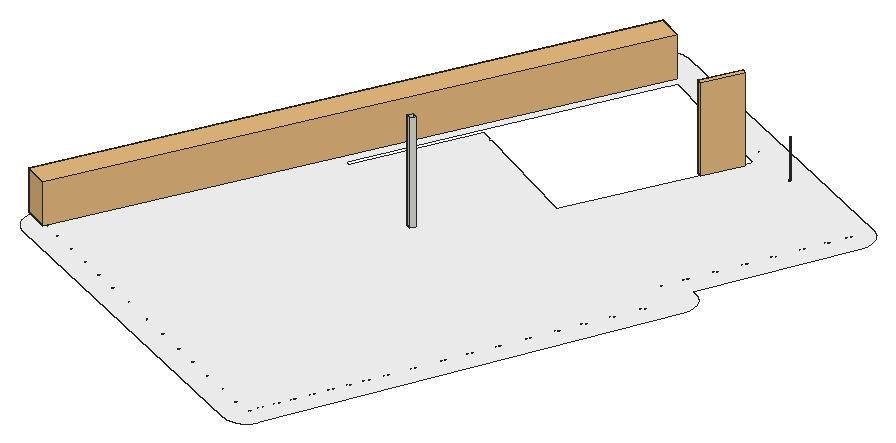
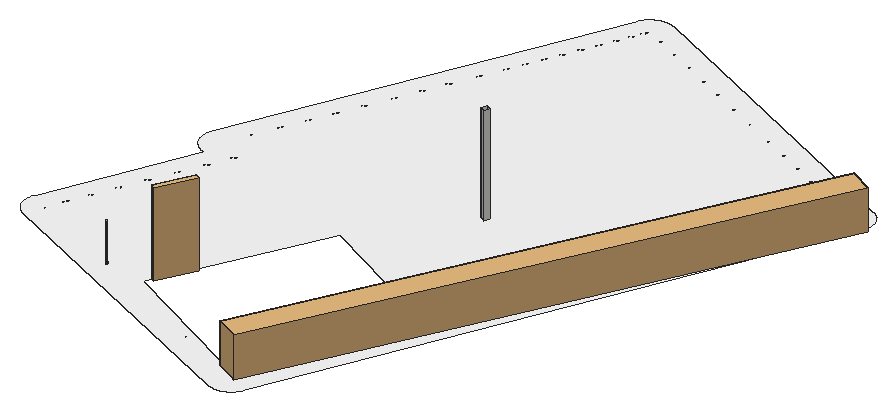
# SketchUp Ruby script. Lengths in inches.
U = 1.inch
M = Sketchup.active_model
def pt(a) = Geom::Point3d.new(a.map { |v| v * U })
def face(e, loops, mat)
  f = e.add_face(loops[0].map { |a| pt(a) })
  loops[1..].each { |l| e.add_face(l.map { |a| pt(a) }).erase! }
  f.material = f.back_material = mat if mat
  f
end
# faces: each face lists its corners as indices into pts; further lists are holes
def faces(e, pts, list, mat = nil) = list.each { |f| face(e, (f[0].is_a?(Array) ? f : [f]).map { |l| l.map { |i| pts[i] } }, mat) }
# xy, xz, yz: faces in a plane at the given z, y or x. An outline is a flat list of corners, or four numbers for a rectangle; further outlines are holes
def ring(l) = l.size == 4 ? [[l[0], l[1]], [l[2], l[1]], [l[2], l[3]], [l[0], l[3]]] : l.each_slice(2).to_a
def flat(e, list, mat, &to3) = list.each { |f| face(e, (f[0].is_a?(Array) ? f : [f]).map { |l| ring(l).map { |u, v| to3.(u, v) } }, mat) }
def xy(e, z, list, mat = nil) = flat(e, list, mat) { |x, y| [x, y, z] }
def xz(e, y, list, mat = nil) = flat(e, list, mat) { |x, z| [x, y, z] }
def yz(e, x, list, mat = nil) = flat(e, list, mat) { |y, z| [x, y, z] }
def lines(e, pts, list) = list.each { |a, b| e.add_line(pt(pts[a]), pt(pts[b])) }
# prism: a flat outline (further loops are holes) pulled along v
def prism(e, loops, v, mat = nil)
  f = face(e, loops, mat); d = Geom::Vector3d.new(v.map { |x| x * U })
  f.pushpull(f.normal.samedirection?(d) ? d.length : -d.length)
end
def box(e, o, s, mat = nil) = prism(e, [[o, [o[0] + s[0], o[1], o[2]], [o[0] + s[0], o[1] + s[1], o[2]], [o[0], o[1] + s[1], o[2]]]], [0, 0, s[2]], mat)
def at(x, y, z, deg = 0) = Geom::Transformation.translation(pt([x, y, z])) * Geom::Transformation.rotation(ORIGIN, Z_AXIS, deg.degrees)
def axes(o, x, y, z) = Geom::Transformation.new([*x, 0, *y, 0, *z, 0, *pt(o).to_a, 1])
def part(name) = M.definitions.add(name)
# library, detail: a bought-in or finely detailed component or shape, given as its bounding box
def library(name, o, s) = part(name).tap { |d| box(d.entities, o, s) }
def detail(e, o, s) = box(e.add_group.entities, o, s)
def put(e, d, t, mat = nil) = e.add_instance(d, t).tap { |i| i.material = mat if mat }
def group(e, t, mat = nil) = e.add_group.tap { |g| g.transformation = t; g.material = mat if mat }.entities
root = M.entities
M.materials.add("[Color_000]").color = [255, 255, 255]
c1 = library("Group\#120",[0,0,0],[510.78,23.69,36.98])
c2 = library("porta 4",[0.2,-5.42,1.33],[46.55,4.72,83.21])
xy(root,321.267,[[[841.443,516.19,840.136,516.256,838.836,516.408,837.549,516.645,836.28,516.965,835.035,517.367,833.818,517.85,548.6875,642.033,547.506,642.595,546.363,643.233,545.264,643.944,544.214,644.725,543.217,645.574,542.279,646.485,541.401,647.457,540.589,648.483,539.846,649.56,539.176,650.684,538.579,651.849,538.061,653.051,537.622,654.284,537.265,655.543,536.991,656.823,536.801,658.118,536.696,659.422,536.677,660.731,536.743,662.038,536.895,663.338,537.132,664.625,537.452,665.894,537.854,667.139,538.337,668.356,741.172,1134.074,741.733,1135.256,742.371,1136.399,743.082,1137.498,743.863,1138.547,744.712,1139.544,745.623,1140.483,746.595,1141.36,747.621,1142.172,748.699,1142.915,749.822,1143.586,750.987,1144.182,752.189,1144.7,753.422,1145.139,754.681,1145.497,755.961,1145.771,757.256,1145.961,758.56,1146.065,759.869,1146.084,761.176,1146.018,762.476,1145.866,763.763,1145.63,765.032,1145.31,766.278,1144.907,767.494,1144.424,1030.621,1029.824,1031.803,1029.263,1032.946,1028.625,1034.045,1027.914,1035.095,1027.133,1036.091,1026.284,1037.03,1025.372,1037.908,1024.401,1038.719,1023.375,1039.462,1022.297,1040.133,1021.174,1040.729,1020.008,1041.248,1018.807,1041.687,1017.574,1042.044,1016.315,1042.318,1015.035,1042.508,1013.74,1042.613,1012.435,1042.632,1011.127,1042.565,1009.82,1042.414,1008.52,1042.177,1007.233,1041.857,1005.964,1041.455,1004.718,1040.971,1003.502,985.468,876.064,989.136,874.467,990.318,873.905,991.461,873.268,992.56,872.556,993.609,871.775,994.606,870.927,995.545,870.015,996.422,869.044,997.234,868.017,997.977,866.94,998.648,865.816,999.244,864.651,999.762,863.449,1000.201,862.216,1000.558,860.957,1000.833,859.677,1001.022,858.382,1001.127,857.078,1001.146,855.769,1001.08,854.462,1000.928,853.162,1000.692,851.875,1000.372,850.606,999.969,849.361,999.486,848.144,860.141,528.201,859.579,527.019,858.942,525.876,858.231,524.777,857.449,523.727,856.601,522.73,855.689,521.792,854.718,520.914,853.691,520.102,852.614,519.359,851.49,518.688,850.325,518.092,849.123,517.574,847.89,517.135,846.631,516.778,845.352,516.504,844.057,516.314,842.752,516.209],[671.218,867.453,718.811,965.468,728.334,960.844,728.204,960.454,728.18,960.044,728.262,959.641,728.446,959.274,728.719,958.966,729.0625,958.74,729.453,958.61,729.863,958.586,730.266,958.668,730.633,958.852,730.941,959.125,731.167,959.469,826.624,913.117,831.121,910.933,881.579,1014.847,896.797,1046.187,897.141,1046.896,900.471,1053.753,783.663,1110.472,780.622,1104.208,780.366,1103.681,780.333,1103.614,714.314,967.652,666.72,869.637],[843.13,535.199,843.291,535.232,843.4375,535.305,843.561,535.415,843.651,535.552,843.703,535.708,843.713,535.872,843.68,536.033,843.606,536.18,843.547,536.247,843.722,536.189,844.132,536.165,844.535,536.247,844.587,536.273,844.902,536.431,845.21,536.704,845.436,537.047,845.566,537.4375,845.59,537.848,845.508,538.251,845.323,538.618,845.051,538.926,844.707,539.152,844.645,539.173,847.388,545.47,847.716,545.361,848.127,545.337,848.529,545.419,848.897,545.603,849.204,545.876,849.431,546.219,849.56,546.61,849.585,547.02,849.502,547.423,849.318,547.79,849.045,548.098,848.702,548.324,848.64,548.345,852.607,557.453,852.935,557.344,853.346,557.32,853.748,557.402,854.116,557.587,854.423,557.859,854.65,558.203,854.78,558.593,854.804,559.003,854.721,559.406,854.537,559.773,854.264,560.081,853.921,560.307,853.859,560.328,858.009,569.857,858.337,569.748,858.748,569.723,859.151,569.806,859.518,569.99,859.826,570.263,860.052,570.606,860.182,570.996,860.206,571.407,860.123,571.809,859.939,572.177,859.666,572.484,859.323,572.711,859.261,572.731,864.264,584.217,864.592,584.108,865.002,584.083,865.405,584.166,865.772,584.35,866.08,584.623,866.306,584.966,866.436,585.356,866.46,585.767,866.378,586.169,866.194,586.537,865.921,586.844,865.577,587.071,865.515,587.091,870.373,598.244,870.701,598.135,871.111,598.11,871.514,598.193,871.882,598.377,872.189,598.65,872.415,598.993,872.545,599.383,872.569,599.794,872.487,600.196,872.303,600.564,872.03,600.871,871.687,601.098,871.625,601.118,876.101,611.396,876.116,611.386,876.506,611.257,876.916,611.232,877.319,611.315,877.687,611.499,877.994,611.772,878.22,612.115,878.35,612.505,878.374,612.916,878.292,613.318,878.108,613.686,877.835,613.993,877.492,614.22,877.351,614.266,882.234,625.478,882.294,625.411,882.637,625.184,883.027,625.055,883.437,625.03,883.84,625.113,884.208,625.297,884.515,625.57,884.741,625.913,884.871,626.303,884.895,626.714,884.813,627.116,884.629,627.484,884.356,627.791,884.013,628.018,883.622,628.147,883.402,628.16,888.589,640.071,888.918,639.961,889.328,639.937,889.731,640.02,890.098,640.204,890.406,640.477,890.632,640.82,890.762,641.21,890.786,641.62,890.704,642.023,890.519,642.391,890.247,642.698,889.903,642.924,889.841,642.945,897.491,660.509,897.819,660.4,898.23,660.376,898.633,660.459,899,660.643,899.308,660.916,899.534,661.259,899.664,661.649,899.688,662.059,899.605,662.462,899.421,662.83,899.148,663.137,898.805,663.363,898.743,663.384,907.436,683.344,907.765,683.235,908.175,683.21,908.578,683.293,908.945,683.477,909.253,683.75,909.479,684.093,909.609,684.483,909.633,684.894,909.55,685.296,909.366,685.664,909.093,685.971,908.75,686.198,908.688,686.218,916.156,703.365,916.484,703.255,916.895,703.231,917.297,703.314,917.665,703.498,917.972,703.771,918.199,704.114,918.328,704.504,918.353,704.914,918.27,705.317,918.086,705.685,917.813,705.992,917.47,706.218,917.408,706.239,925.387,724.56,925.716,724.451,926.126,724.427,926.529,724.51,926.896,724.694,927.204,724.967,927.43,725.31,927.56,725.7,927.584,726.11,927.501,726.513,927.317,726.881,927.044,727.188,926.701,727.414,926.639,727.435,935.3125,747.349,935.641,747.24,936.051,747.215,936.454,747.298,936.821,747.482,937.129,747.755,937.355,748.098,937.485,748.488,937.509,748.899,937.426,749.301,937.242,749.669,936.969,749.976,936.626,750.203,936.564,750.223,944.632,768.748,944.647,768.738,945.037,768.608,945.448,768.584,945.85,768.666,946.218,768.85,946.525,769.123,946.752,769.467,946.881,769.857,946.906,770.267,946.823,770.67,946.639,771.037,946.366,771.345,946.023,771.571,945.882,771.618,953.644,789.44,953.917,789.133,954.261,788.907,954.651,788.777,955.061,788.753,955.464,788.835,955.831,789.019,956.139,789.292,956.365,789.636,956.495,790.026,956.519,790.436,956.437,790.839,956.252,791.206,955.979,791.514,955.636,791.74,955.246,791.87,954.836,791.894,954.701,791.867,962.796,810.452,963.124,810.343,963.534,810.319,963.937,810.401,964.305,810.585,964.612,810.858,964.838,811.202,964.968,811.592,964.993,812.002,964.91,812.405,964.726,812.772,964.453,813.08,964.11,813.306,964.048,813.327,972.962,833.794,973.29,833.685,973.7,833.66,974.103,833.743,974.471,833.927,974.778,834.2,975.004,834.543,975.134,834.933,975.159,835.344,975.076,835.746,974.892,836.114,974.619,836.421,974.276,836.648,974.214,836.668,973.886,836.777,973.475,836.802,973.072,836.719,972.705,836.535,972.397,836.262,972.171,835.919,972.041,835.529,972.017,835.118,972.1,834.716,972.284,834.348,972.557,834.041,972.9,833.814,972.962,833.794,964.048,813.327,963.72,813.436,963.309,813.46,962.906,813.377,962.539,813.193,962.231,812.92,962.005,812.577,961.875,812.187,961.851,811.777,961.934,811.374,962.118,811.006,962.391,810.699,962.734,810.473,962.796,810.452,954.701,791.867,954.433,791.811,954.065,791.627,953.758,791.354,953.532,791.011,953.402,790.621,953.378,790.211,953.46,789.808,953.644,789.44,945.882,771.618,945.633,771.701,945.222,771.725,944.82,771.643,944.452,771.458,944.145,771.185,943.918,770.842,943.789,770.452,943.764,770.042,943.847,769.639,944.031,769.272,944.304,768.964,944.632,768.748,936.564,750.223,936.236,750.332,935.826,750.357,935.423,750.274,935.055,750.09,934.748,749.817,934.522,749.474,934.392,749.084,934.368,748.673,934.45,748.271,934.634,747.903,934.907,747.596,935.251,747.369,935.3125,747.349,926.639,727.435,926.311,727.544,925.901,727.568,925.498,727.486,925.13,727.302,924.823,727.029,924.597,726.686,924.467,726.295,924.443,725.885,924.525,725.482,924.709,725.115,924.982,724.807,925.325,724.581,925.387,724.56,917.408,706.239,917.08,706.348,916.669,706.373,916.267,706.29,915.899,706.106,915.592,705.833,915.365,705.49,915.236,705.1,915.211,704.689,915.294,704.287,915.478,703.919,915.751,703.612,916.094,703.385,916.156,703.365,908.688,686.218,908.36,686.327,907.95,686.352,907.547,686.269,907.179,686.085,906.872,685.812,906.646,685.469,906.516,685.079,906.492,684.668,906.574,684.266,906.758,683.898,907.031,683.591,907.374,683.364,907.436,683.344,898.743,663.384,898.415,663.493,898.005,663.517,897.602,663.435,897.234,663.251,896.927,662.978,896.701,662.635,896.571,662.245,896.546,661.834,896.629,661.431,896.813,661.064,897.086,660.756,897.429,660.53,897.491,660.509,889.841,642.945,889.513,643.054,889.103,643.079,888.7,642.996,888.333,642.812,888.025,642.539,887.799,642.196,887.669,641.806,887.645,641.395,887.727,640.992,887.911,640.625,888.184,640.317,888.528,640.091,888.589,640.071,883.402,628.16,883.212,628.172,882.809,628.089,882.442,627.905,882.134,627.632,881.908,627.289,881.778,626.899,881.754,626.488,881.837,626.086,882.021,625.718,882.234,625.478,877.351,614.266,877.101,614.349,876.691,614.374,876.288,614.291,875.921,614.107,875.613,613.834,875.387,613.491,875.257,613.101,875.233,612.69,875.316,612.288,875.5,611.92,875.773,611.613,876.101,611.396,871.625,601.118,871.296,601.227,870.886,601.252,870.483,601.169,870.116,600.985,869.808,600.712,869.582,600.369,869.452,599.979,869.428,599.568,869.511,599.166,869.695,598.798,869.968,598.491,870.311,598.264,870.373,598.244,865.515,587.091,865.187,587.2,864.777,587.225,864.374,587.142,864.007,586.958,863.699,586.685,863.473,586.342,863.343,585.952,863.319,585.541,863.401,585.139,863.585,584.771,863.858,584.464,864.202,584.237,864.264,584.217,859.261,572.731,858.933,572.84,858.523,572.865,858.12,572.782,857.752,572.598,857.445,572.325,857.219,571.982,857.089,571.592,857.065,571.181,857.147,570.779,857.331,570.411,857.604,570.104,857.947,569.877,858.009,569.857,853.859,560.328,853.531,560.437,853.121,560.461,852.718,560.379,852.35,560.195,852.043,559.922,851.817,559.578,851.687,559.188,851.662,558.778,851.745,558.375,851.929,558.008,852.202,557.7,852.545,557.474,852.607,557.453,848.64,548.345,848.312,548.454,847.902,548.478,847.499,548.395,847.131,548.211,846.824,547.938,846.597,547.595,846.468,547.205,846.443,546.795,846.526,546.392,846.71,546.024,846.983,545.717,847.326,545.491,847.388,545.47,844.645,539.173,844.317,539.282,843.907,539.306,843.504,539.223,843.137,539.039,842.829,538.766,842.603,538.423,842.473,538.033,842.449,537.623,842.517,537.289,842.531,537.22,842.715,536.852,842.988,536.545,843.133,536.45,843.039,536.455,842.878,536.422,842.731,536.349,842.608,536.239,842.518,536.102,842.466,535.946,842.456,535.782,842.489,535.621,842.563,535.474,842.672,535.351,842.809,535.26,842.846,535.248,842.965,535.208],[827.381,539.408,827.783,539.491,828.151,539.675,828.458,539.948,828.685,540.291,828.705,540.352,828.815,540.681,828.839,541.092,828.756,541.494,828.572,541.862,828.299,542.169,827.956,542.396,827.566,542.525,827.156,542.55,826.753,542.467,826.385,542.283,826.078,542.01,825.851,541.667,825.83,541.603,809.71,548.624,809.819,548.953,809.844,549.363,809.761,549.766,809.577,550.133,809.304,550.441,808.961,550.667,808.571,550.797,808.16,550.821,807.758,550.738,807.39,550.554,807.083,550.281,806.856,549.938,806.836,549.876,788.49,557.867,788.599,558.195,788.623,558.605,788.54,559.008,788.356,559.375,788.083,559.683,787.74,559.909,787.35,560.039,786.94,560.063,786.537,559.981,786.169,559.797,785.862,559.524,785.636,559.18,785.615,559.118,767.513,567.002,767.623,567.33,767.647,567.741,767.564,568.144,767.38,568.511,767.107,568.819,766.764,569.045,766.374,569.175,765.964,569.199,765.561,569.116,765.193,568.932,764.886,568.659,764.66,568.316,764.639,568.254,747.167,575.864,747.276,576.192,747.301,576.602,747.218,577.005,747.034,577.373,746.761,577.68,746.418,577.906,746.028,578.036,745.617,578.06,745.215,577.978,744.847,577.794,744.54,577.521,744.313,577.178,744.293,577.116,724.462,585.753,724.571,586.081,724.596,586.491,724.513,586.894,724.329,587.261,724.056,587.569,723.713,587.795,723.323,587.925,722.912,587.949,722.509,587.867,722.142,587.682,721.834,587.41,721.608,587.066,721.588,587.004,701.946,595.559,702.055,595.887,702.08,596.297,701.997,596.7,701.813,597.068,701.54,597.375,701.197,597.601,700.807,597.731,700.396,597.756,699.994,597.673,699.626,597.489,699.319,597.216,699.092,596.873,699.072,596.811,675.709,606.986,675.818,607.314,675.843,607.724,675.76,608.127,675.576,608.495,675.303,608.802,674.96,609.028,674.57,609.158,674.159,609.183,673.757,609.1,673.389,608.916,673.082,608.643,672.855,608.3,672.835,608.238,653.14,616.816,653.249,617.144,653.273,617.554,653.19,617.957,653.006,618.324,652.733,618.632,652.39,618.858,652,618.988,651.59,619.012,651.187,618.93,650.819,618.746,650.512,618.473,650.286,618.129,650.265,618.067,633.494,625.372,633.603,625.7,633.628,626.11,633.545,626.513,633.361,626.881,633.088,627.188,632.745,627.414,632.355,627.544,631.944,627.568,631.542,627.486,631.174,627.302,630.867,627.029,630.64,626.686,630.62,626.624,613.859,633.924,613.968,634.252,613.992,634.662,613.91,635.065,613.726,635.432,613.453,635.74,613.109,635.966,612.719,636.096,612.309,636.12,611.906,636.038,611.539,635.854,611.231,635.581,611.005,635.237,610.984,635.175,593.863,642.632,593.972,642.961,593.996,643.371,593.914,643.774,593.73,644.141,593.457,644.449,593.113,644.675,592.723,644.805,592.313,644.829,591.91,644.746,591.543,644.5625,591.235,644.289,591.009,643.946,590.988,643.884,574.051,651.261,574.16,651.589,574.184,652,574.101,652.402,573.917,652.77,573.644,653.077,573.301,653.304,572.911,653.434,572.501,653.458,572.098,653.375,571.73,653.191,571.423,652.918,571.197,652.575,571.176,652.513,558.139,658.191,558.27,658.307,558.496,658.65,558.626,659.04,558.65,659.451,558.568,659.854,558.383,660.221,558.111,660.529,557.767,660.755,557.377,660.885,556.967,660.909,556.564,660.826,556.197,660.642,555.901,660.38,555.889,660.369,555.663,660.026,555.533,659.636,555.529,659.561,555.509,659.226,555.591,658.823,555.775,658.455,555.88,658.337,556.048,658.148,556.392,657.922,556.782,657.792,557.192,657.767,557.595,657.85,557.962,658.034,558.139,658.191,571.176,652.513,571.067,652.185,571.043,651.775,571.125,651.372,571.309,651.004,571.582,650.697,571.925,650.471,572.316,650.341,572.726,650.316,573.129,650.399,573.496,650.583,573.804,650.856,574.03,651.199,574.051,651.261,590.988,643.884,590.879,643.556,590.855,643.146,590.9375,642.743,591.121,642.375,591.394,642.068,591.738,641.842,592.128,641.712,592.538,641.6875,592.941,641.77,593.308,641.954,593.616,642.227,593.842,642.57,593.863,642.632,610.984,635.175,610.875,634.847,610.851,634.437,610.933,634.034,611.117,633.667,611.39,633.359,611.734,633.133,612.124,633.003,612.534,632.979,612.937,633.061,613.304,633.245,613.612,633.518,613.838,633.862,613.859,633.924,630.62,626.624,630.511,626.295,630.486,625.885,630.569,625.482,630.753,625.115,631.026,624.807,631.369,624.581,631.759,624.451,632.17,624.427,632.572,624.51,632.94,624.694,633.247,624.967,633.474,625.31,633.494,625.372,650.265,618.067,650.156,617.739,650.132,617.329,650.214,616.926,650.398,616.559,650.671,616.251,651.014,616.025,651.405,615.895,651.815,615.871,652.218,615.953,652.585,616.138,652.893,616.41,653.119,616.754,653.14,616.816,672.835,608.238,672.726,607.91,672.701,607.499,672.784,607.096,672.968,606.729,673.241,606.421,673.584,606.195,673.974,606.065,674.385,606.041,674.787,606.124,675.155,606.308,675.462,606.581,675.689,606.924,675.709,606.986,699.072,596.811,698.962,596.483,698.938,596.072,699.021,595.67,699.205,595.302,699.478,594.994,699.821,594.768,700.211,594.638,700.621,594.614,701.024,594.697,701.392,594.881,701.699,595.154,701.925,595.497,701.946,595.559,721.588,587.004,721.478,586.676,721.454,586.266,721.537,585.863,721.721,585.496,721.994,585.188,722.337,584.962,722.727,584.832,723.137,584.808,723.54,584.89,723.908,585.074,724.215,585.347,724.441,585.691,724.462,585.753,744.293,577.116,744.184,576.787,744.159,576.377,744.242,575.974,744.426,575.607,744.699,575.299,745.042,575.073,745.432,574.943,745.843,574.919,746.245,575.002,746.613,575.186,746.92,575.459,747.147,575.802,747.167,575.864,764.639,568.254,764.53,567.926,764.505,567.516,764.588,567.113,764.772,566.745,765.045,566.438,765.388,566.212,765.778,566.082,766.189,566.057,766.592,566.14,766.959,566.324,767.267,566.597,767.493,566.94,767.513,567.002,785.615,559.118,785.506,558.79,785.482,558.38,785.564,557.977,785.748,557.61,786.021,557.302,786.364,557.076,786.755,556.946,787.165,556.922,787.568,557.004,787.935,557.188,788.243,557.461,788.469,557.805,788.49,557.867,806.836,549.876,806.726,549.548,806.702,549.138,806.785,548.735,806.969,548.367,807.242,548.06,807.585,547.834,807.975,547.704,808.385,547.68,808.788,547.762,809.156,547.946,809.463,548.219,809.69,548.5625,809.71,548.624,825.83,541.603,825.722,541.277,825.697,540.866,825.78,540.464,825.964,540.096,826.237,539.789,826.58,539.5625,826.97,539.433],[961.916,866.707,962.319,866.79,962.686,866.974,962.994,867.247,963.22,867.59,963.35,867.98,963.374,868.391,963.291,868.793,963.107,869.161,962.834,869.469,962.491,869.695,962.429,869.715,970.135,887.408,970.463,887.298,970.873,887.274,971.276,887.357,971.644,887.541,971.951,887.814,972.177,888.157,972.307,888.547,972.332,888.957,972.249,889.36,972.065,889.728,971.792,890.035,971.449,890.261,971.387,890.282,979.763,909.514,980.091,909.405,980.502,909.381,980.904,909.464,981.272,909.648,981.579,909.921,981.806,910.264,981.935,910.654,981.96,911.064,981.877,911.467,981.693,911.835,981.42,912.142,981.077,912.368,981.015,912.389,989.406,931.655,989.734,931.545,990.144,931.521,990.547,931.604,990.915,931.788,991.222,932.061,991.448,932.404,991.578,932.794,991.602,933.204,991.52,933.607,991.336,933.975,991.063,934.282,990.72,934.508,990.658,934.529,999.023,953.736,999.351,953.627,999.761,953.602,1000.164,953.685,1000.532,953.869,1000.839,954.142,1001.065,954.485,1001.195,954.875,1001.219,955.286,1001.137,955.688,1000.953,956.056,1000.68,956.363,1000.337,956.59,1000.275,956.61,1008.368,975.194,1008.696,975.085,1009.107,975.06,1009.51,975.143,1009.877,975.327,1010.185,975.6,1010.411,975.943,1010.541,976.333,1010.565,976.744,1010.482,977.146,1010.298,977.514,1010.025,977.821,1009.682,978.048,1009.62,978.068,1016.34,993.498,1016.669,993.389,1017.079,993.365,1017.482,993.447,1017.849,993.631,1018.157,993.904,1018.383,994.248,1018.513,994.638,1018.537,995.048,1018.455,995.451,1018.27,995.818,1017.998,996.126,1017.654,996.352,1017.592,996.373,1023.808,1010.645,1023.955,1011.013,1023.974,1011.074,1023.991,1011.073,1024.394,1011.156,1024.762,1011.34,1025.069,1011.613,1025.295,1011.956,1025.425,1012.346,1025.45,1012.756,1025.367,1013.159,1025.183,1013.527,1024.91,1013.834,1024.567,1014.061,1024.177,1014.19,1023.766,1014.215,1023.363,1014.132,1023.238,1014.069,1022.996,1013.948,1022.688,1013.675,1022.538,1013.446,1022.462,1013.332,1022.396,1013.133,1022.332,1012.942,1022.308,1012.531,1022.32,1012.471,1022.391,1012.129,1022.575,1011.761,1022.704,1011.616,1022.848,1011.454,1023.191,1011.227,1023.581,1011.098,1023.974,1011.074,1023.955,1011.013,1023.808,1010.645,1017.592,996.373,1017.264,996.482,1016.854,996.506,1016.451,996.424,1016.084,996.24,1015.776,995.967,1015.55,995.623,1015.42,995.233,1015.396,994.823,1015.478,994.42,1015.662,994.053,1015.935,993.745,1016.279,993.519,1016.34,993.498,1009.62,978.068,1009.292,978.177,1008.882,978.202,1008.479,978.119,1008.111,977.935,1007.804,977.662,1007.578,977.319,1007.448,976.929,1007.423,976.518,1007.506,976.116,1007.69,975.748,1007.963,975.441,1008.306,975.214,1008.368,975.194,1000.275,956.61,999.946,956.719,999.536,956.744,999.133,956.661,998.766,956.477,998.458,956.204,998.232,955.861,998.102,955.471,998.078,955.06,998.161,954.658,998.345,954.29,998.618,953.983,998.961,953.756,999.023,953.736,990.658,934.529,990.329,934.638,989.919,934.663,989.516,934.58,989.149,934.396,988.841,934.123,988.615,933.78,988.485,933.39,988.461,932.979,988.544,932.577,988.728,932.209,989.001,931.901,989.344,931.675,989.406,931.655,981.015,912.389,980.687,912.498,980.276,912.522,979.874,912.44,979.506,912.256,979.199,911.983,978.972,911.64,978.843,911.249,978.818,910.839,978.901,910.436,979.085,910.069,979.358,909.761,979.701,909.535,979.763,909.514,971.387,890.282,971.059,890.391,970.648,890.416,970.245,890.333,969.878,890.149,969.57,889.876,969.344,889.533,969.214,889.143,969.19,888.732,969.273,888.33,969.457,887.962,969.73,887.655,970.073,887.428,970.135,887.408,962.429,869.715,962.101,869.825,961.691,869.849,961.288,869.766,960.92,869.582,960.613,869.309,960.387,868.966,960.257,868.576,960.233,868.166,960.315,867.763,960.499,867.395,960.772,867.088,961.115,866.862,961.177,866.841,961.506,866.732],[765.123,821.855,767.291,826.319,762.793,828.503,760.626,824.039],[554.814,657.808,555.217,657.891,555.585,658.075,555.88,658.337,555.892,658.348,556.118,658.691,556.231,659.029,556.248,659.081,556.273,659.492,556.19,659.894,556.006,660.262,555.901,660.38,555.733,660.569,555.39,660.796,555.343,660.811,555,660.925,554.589,660.95,554.186,660.867,553.819,660.683,553.511,660.41,553.285,660.067,553.155,659.677,553.131,659.266,553.214,658.864,553.398,658.496,553.671,658.189,554.014,657.962,554.404,657.833],[824.098,1097.975,824.501,1098.058,824.868,1098.242,825.176,1098.515,825.402,1098.858,825.423,1098.92,824.56,1099.296,824.604,1099.427,824.614,1099.591,824.581,1099.752,824.507,1099.899,824.398,1100.022,824.261,1100.113,824.105,1100.165,823.94,1100.175,823.779,1100.142,823.632,1100.068,823.509,1099.959,823.419,1099.821,823.411,1099.797,822.548,1100.172,822.439,1099.844,822.415,1099.434,822.497,1099.031,822.681,1098.663,822.954,1098.356,823.298,1098.13,823.6875,1098],[1015.608,1014.567,1016.011,1014.65,1016.378,1014.834,1016.686,1015.107,1016.912,1015.45,1016.932,1015.512,1016.07,1015.888,1016.114,1016.019,1016.124,1016.183,1016.09,1016.344,1016.017,1016.491,1015.908,1016.614,1015.77,1016.705,1015.614,1016.757,1015.45,1016.766,1015.289,1016.733,1015.142,1016.66,1015.019,1016.55,1014.929,1016.413,1014.92,1016.388,1014.058,1016.764,1013.949,1016.436,1013.924,1016.025,1014.007,1015.623,1014.191,1015.255,1014.464,1014.948,1014.807,1014.721,1015.197,1014.592],[871.348,1077.397,871.751,1077.479,872.118,1077.663,872.426,1077.936,872.652,1078.28,872.673,1078.342,871.81,1078.717,871.854,1078.848,871.864,1079.013,871.831,1079.174,871.757,1079.321,871.648,1079.444,871.511,1079.534,871.355,1079.586,871.19,1079.596,871.029,1079.563,870.882,1079.489,870.759,1079.38,870.669,1079.243,870.661,1079.218,869.798,1079.593,869.689,1079.265,869.665,1078.855,869.747,1078.452,869.931,1078.085,870.204,1077.777,870.548,1077.551,870.9375,1077.421],[893.192,1067.883,893.595,1067.966,893.962,1068.15,894.27,1068.423,894.496,1068.766,894.517,1068.828,893.654,1069.203,893.698,1069.335,893.708,1069.499,893.675,1069.66,893.601,1069.807,893.492,1069.93,893.354,1070.02,893.198,1070.072,893.034,1070.082,892.873,1070.049,892.726,1069.975,892.603,1069.866,892.513,1069.729,892.504,1069.704,891.642,1070.08,891.533,1069.752,891.509,1069.341,891.591,1068.938,891.775,1068.571,892.048,1068.263,892.391,1068.037,892.782,1067.907],[916.821,1057.592,917.223,1057.675,917.591,1057.859,917.898,1058.132,918.125,1058.475,918.145,1058.537,917.283,1058.912,917.327,1059.044,917.336,1059.208,917.303,1059.369,917.23,1059.516,917.121,1059.639,916.983,1059.729,916.827,1059.781,916.663,1059.791,916.502,1059.758,916.355,1059.684,916.232,1059.575,916.142,1059.438,916.133,1059.413,915.271,1059.789,915.162,1059.461,915.137,1059.05,915.22,1058.647,915.404,1058.28,915.677,1057.972,916.02,1057.746,916.41,1057.616],[938.054,1048.344,938.457,1048.427,938.824,1048.611,939.132,1048.884,939.358,1049.227,939.379,1049.289,938.516,1049.665,938.56,1049.796,938.57,1049.96,938.537,1050.121,938.463,1050.268,938.354,1050.391,938.217,1050.482,938.061,1050.534,937.896,1050.543,937.735,1050.51,937.588,1050.437,937.465,1050.327,937.375,1050.19,937.367,1050.165,936.504,1050.541,936.395,1050.213,936.371,1049.802,936.453,1049.4,936.637,1049.032,936.91,1048.725,937.254,1048.498,937.644,1048.369],[957.437,1039.902,957.84,1039.985,958.208,1040.169,958.515,1040.442,958.741,1040.785,958.762,1040.847,957.9,1041.223,957.943,1041.354,957.953,1041.518,957.92,1041.679,957.846,1041.826,957.737,1041.949,957.6,1042.04,957.444,1042.092,957.28,1042.101,957.118,1042.068,956.971,1041.995,956.848,1041.885,956.758,1041.748,956.75,1041.723,955.887,1042.099,955.778,1041.771,955.754,1041.36,955.837,1040.958,956.021,1040.59,956.294,1040.283,956.637,1040.056,957.027,1039.927],[800.488,1108.258,800.891,1108.341,801.258,1108.525,801.566,1108.798,801.792,1109.141,801.813,1109.203,800.95,1109.579,800.994,1109.71,801.004,1109.874,800.971,1110.035,800.897,1110.182,800.788,1110.305,800.651,1110.396,800.495,1110.448,800.331,1110.457,800.169,1110.424,800.022,1110.351,799.899,1110.242,799.809,1110.104,799.801,1110.079,798.938,1110.455,798.829,1110.127,798.805,1109.716,798.887,1109.314,799.072,1108.946,799.344,1108.639,799.6875,1108.412,800.078,1108.283],[996.475,1022.9,996.878,1022.983,997.246,1023.167,997.553,1023.44,997.779,1023.783,997.8,1023.845,996.938,1024.22,996.981,1024.352,996.991,1024.516,996.958,1024.677,996.884,1024.824,996.775,1024.947,996.638,1025.037,996.482,1025.089,996.318,1025.099,996.157,1025.066,996.01,1024.992,995.887,1024.883,995.796,1024.746,995.788,1024.721,994.926,1025.097,994.816,1024.769,994.792,1024.358,994.875,1023.955,995.059,1023.588,995.332,1023.28,995.675,1023.054,996.065,1022.924],[975.893,1031.864,976.296,1031.947,976.663,1032.131,976.971,1032.404,977.197,1032.747,977.218,1032.809,976.355,1033.185,976.399,1033.316,976.409,1033.48,976.376,1033.641,976.302,1033.788,976.193,1033.911,976.056,1034.002,975.9,1034.054,975.735,1034.063,975.574,1034.03,975.427,1033.957,975.304,1033.847,975.214,1033.71,975.206,1033.685,974.343,1034.061,974.234,1033.733,974.21,1033.322,974.292,1032.92,974.476,1032.552,974.749,1032.245,975.093,1032.018,975.483,1031.889],[848.682,1087.269,849.084,1087.351,849.452,1087.535,849.759,1087.808,849.986,1088.151,850.006,1088.213,849.144,1088.589,849.1875,1088.72,849.197,1088.884,849.164,1089.045,849.091,1089.192,848.982,1089.315,848.844,1089.406,848.688,1089.458,848.524,1089.468,848.363,1089.435,848.216,1089.361,848.093,1089.252,848.002,1089.114,847.994,1089.09,847.132,1089.465,847.023,1089.137,846.998,1088.727,847.081,1088.324,847.265,1087.956,847.538,1087.649,847.881,1087.423,848.271,1087.293],[760.58,1127.161,760.587,1127.184,760.612,1127.594,760.529,1127.997,760.345,1128.364,760.072,1128.672,759.729,1128.898,759.339,1129.028,758.929,1129.052,758.526,1128.969,758.158,1128.785,757.851,1128.512,757.624,1128.169,757.495,1127.779,757.483,1127.574,757.641,1127.607,758.052,1127.582,758.414,1127.462,758.423,1127.6,758.474,1127.756,758.565,1127.894,758.688,1128.003,758.835,1128.077,758.996,1128.11,759.16,1128.1,759.316,1128.048,759.454,1127.957,759.563,1127.834,759.636,1127.6875,759.669,1127.526,759.667,1127.48,759.716,1127.475,759.806,1127.458,759.895,1127.436,759.983,1127.407,760.351,1127.261],[776.144,1118.861,776.547,1118.944,776.914,1119.128,777.222,1119.401,777.448,1119.744,777.469,1119.806,776.606,1120.181,776.598,1120.156,776.508,1120.019,776.385,1119.91,776.238,1119.836,776.077,1119.803,775.912,1119.813,775.756,1119.865,775.619,1119.956,775.51,1120.078,775.436,1120.226,775.403,1120.387,775.413,1120.551,775.457,1120.682,774.594,1121.058,774.485,1120.729,774.461,1120.319,774.543,1119.916,774.728,1119.549,775,1119.241,775.344,1119.015,775.734,1118.885],[982.5,856.655,982.661,856.688,982.808,856.762,982.931,856.871,983.022,857.008,983.074,857.164,983.083,857.328,983.05,857.489,982.977,857.636,982.868,857.759,982.73,857.85,982.574,857.902,982.41,857.912,982.249,857.878,982.136,857.822,982.102,857.805,981.979,857.696,981.888,857.558,981.837,857.402,981.834,857.354,981.827,857.238,981.86,857.077,981.934,856.93,982.004,856.851,982.043,856.807,982.18,856.717,982.336,856.665,982.449,856.658],[1022.108,1012.412,1022.269,1012.445,1022.32,1012.471,1022.416,1012.519,1022.539,1012.628,1022.63,1012.766,1022.681,1012.922,1022.686,1013.006,1022.691,1013.086,1022.658,1013.247,1022.584,1013.394,1022.538,1013.446,1022.475,1013.517,1022.338,1013.607,1022.182,1013.659,1022.018,1013.669,1021.857,1013.636,1021.71,1013.562,1021.611,1013.474,1021.587,1013.453,1021.496,1013.316,1021.444,1013.16,1021.435,1012.996,1021.468,1012.835,1021.541,1012.6875,1021.65,1012.565,1021.788,1012.474,1021.944,1012.422],[980.642,856.926,980.803,856.959,980.916,857.016,980.95,857.033,981.073,857.142,981.164,857.279,981.216,857.435,981.225,857.599,981.217,857.642,981.192,857.76,981.119,857.907,981.049,857.986,981.01,858.03,980.872,858.121,980.716,858.173,980.552,858.183,980.391,858.15,980.244,858.076,980.236,858.069,980.121,857.967,980.03,857.829,979.979,857.673,979.969,857.509,980.002,857.348,980.075,857.201,980.185,857.078,980.322,856.988,980.478,856.936],[759.154,1125.911,759.3125,1125.943,759.325,1126.148,759.242,1126.551,759.09,1126.854,759.086,1126.853,758.922,1126.863,758.766,1126.915,758.629,1127.005,758.541,1127.103,758.534,1127.097,758.47,1127.031,758.411,1126.961,758.356,1126.888,758.306,1126.811,758.262,1126.731,758.16,1126.516,758.166,1126.512,758.276,1126.389,758.349,1126.242,758.382,1126.081,758.381,1126.056,758.743,1125.935],[776.606,1120.181,776.65,1120.3125,776.66,1120.477,776.627,1120.638,776.553,1120.785,776.444,1120.908,776.307,1120.998,776.151,1121.05,775.987,1121.06,775.825,1121.027,775.678,1120.953,775.555,1120.844,775.465,1120.707,775.457,1120.682],[800.421,1109.201,800.582,1109.234,800.729,1109.307,800.852,1109.417,800.942,1109.554,800.95,1109.579,799.801,1110.079,799.757,1109.948,799.747,1109.784,799.78,1109.623,799.854,1109.476,799.963,1109.353,800.1,1109.262,800.256,1109.211],[1015.54,1015.51,1015.701,1015.543,1015.848,1015.616,1015.971,1015.726,1016.062,1015.863,1016.07,1015.888,1014.92,1016.388,1014.877,1016.257,1014.867,1016.093,1014.9,1015.932,1014.974,1015.785,1015.083,1015.662,1015.22,1015.571,1015.376,1015.519],[871.28,1078.339,871.442,1078.372,871.589,1078.446,871.712,1078.555,871.802,1078.692,871.81,1078.717,870.661,1079.218,870.617,1079.087,870.607,1078.922,870.64,1078.761,870.714,1078.614,870.823,1078.491,870.96,1078.401,871.116,1078.349],[996.408,1023.842,996.569,1023.875,996.716,1023.949,996.839,1024.058,996.929,1024.196,996.938,1024.22,995.788,1024.721,995.744,1024.59,995.735,1024.426,995.768,1024.265,995.841,1024.118,995.95,1023.995,996.088,1023.904,996.244,1023.852],[975.826,1032.807,975.987,1032.84,976.134,1032.913,976.257,1033.023,976.347,1033.16,976.355,1033.185,975.206,1033.685,975.162,1033.554,975.152,1033.39,975.185,1033.229,975.259,1033.082,975.368,1032.959,975.505,1032.868,975.661,1032.816],[848.614,1088.211,848.775,1088.244,848.922,1088.318,849.045,1088.427,849.136,1088.564,849.144,1088.589,847.994,1089.09,847.951,1088.958,847.941,1088.794,847.974,1088.633,848.048,1088.486,848.157,1088.363,848.294,1088.273,848.45,1088.221],[937.987,1049.287,938.148,1049.32,938.295,1049.393,938.418,1049.503,938.508,1049.64,938.516,1049.665,937.367,1050.165,937.323,1050.034,937.313,1049.87,937.346,1049.709,937.42,1049.562,937.529,1049.439,937.666,1049.348,937.822,1049.296],[916.753,1058.534,916.914,1058.567,917.061,1058.641,917.184,1058.75,917.275,1058.888,917.283,1058.912,916.133,1059.413,916.09,1059.282,916.08,1059.118,916.113,1058.957,916.187,1058.81,916.296,1058.687,916.433,1058.596,916.589,1058.544],[759.09,1126.854,759.247,1126.886,759.394,1126.96,759.517,1127.069,759.608,1127.206,759.66,1127.362,759.667,1127.48,759.625,1127.485,759.533,1127.49,759.442,1127.488,759.35,1127.481,759.259,1127.468,759.17,1127.449,759.081,1127.424,758.995,1127.393,758.911,1127.356,758.829,1127.315,758.75,1127.268,758.736,1127.258,758.785,1127.226,759.058,1126.919],[758.046,1126.267,758.092,1126.373,758.16,1126.516,758.029,1126.602,757.873,1126.654,757.709,1126.664,757.705,1126.663,757.737,1126.598,758.01,1126.291],[758.541,1127.103,758.602,1127.159,758.674,1127.216,758.736,1127.258,758.442,1127.452,758.414,1127.462,758.413,1127.436,758.446,1127.275,758.519,1127.128],[843.547,536.247,843.497,536.303,843.418,536.355,843.36,536.394,843.204,536.446,843.133,536.45,843.332,536.319,843.393,536.298]],[765.123,821.855,760.626,824.039,762.793,828.503,767.291,826.319]],"[Color_000]")
p = [[765.123,821.855,321.267],[765.123,821.855,412.837],[760.626,824.039,412.837],[760.626,824.039,321.267],[767.291,826.319,321.267],[767.291,826.319,412.837],
  [762.793,828.503,321.267],[762.793,828.503,412.837],[937.254,1048.498,321.267],[937.644,1048.369,321.267],[937.644,1048.369,321.858],[937.254,1048.498,321.858],
  [936.91,1048.725,321.267],[936.91,1048.725,321.858],[936.637,1049.032,321.267],[936.637,1049.032,321.858],[936.453,1049.4,321.267],[936.453,1049.4,321.858],
  [937.529,1049.439,321.267],[937.666,1049.348,321.267],[937.666,1049.348,357.267],[937.529,1049.439,357.267],[937.822,1049.296,321.267],[937.822,1049.296,357.267],
  [936.371,1049.802,321.267],[936.371,1049.802,321.858],[937.42,1049.562,321.267],[937.42,1049.562,357.267],[937.346,1049.709,321.267],[937.346,1049.709,357.267],
  [937.313,1049.87,321.267],[937.313,1049.87,357.267],[936.395,1050.213,321.267],[936.395,1050.213,321.858],[937.323,1050.034,321.267],[937.323,1050.034,357.267]]
faces(root,p,[[0,1,2,3],[0,4,5,1],[6,3,2,7],[5,4,6,7],[8,9,10,11],[12,8,11,13],[14,12,13,15],[16,14,15,17],
  [24,16,17,25],[32,24,25,33]])
faces(root,p,[[18,19,20,21],[19,22,23,20],[26,18,21,27],[28,26,27,29],[30,28,29,31],[34,30,31,35]],"[Color_000]")
put(root,c1,at(555.24,656.89,321.27,64.1))
put(root,c2,axes([877.46,1016.75,320.01],[0.33912,0.6854,0],[-0.89629,0.44347,0],[0,0,0.93749]))
